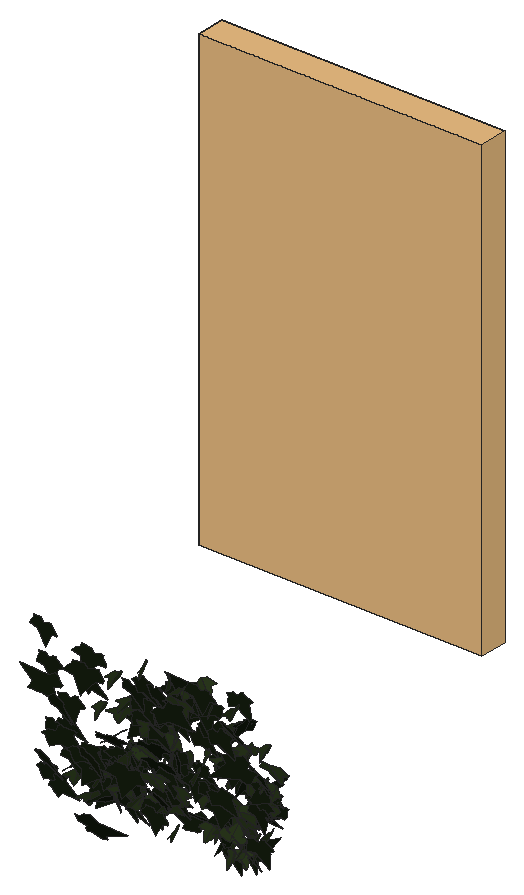
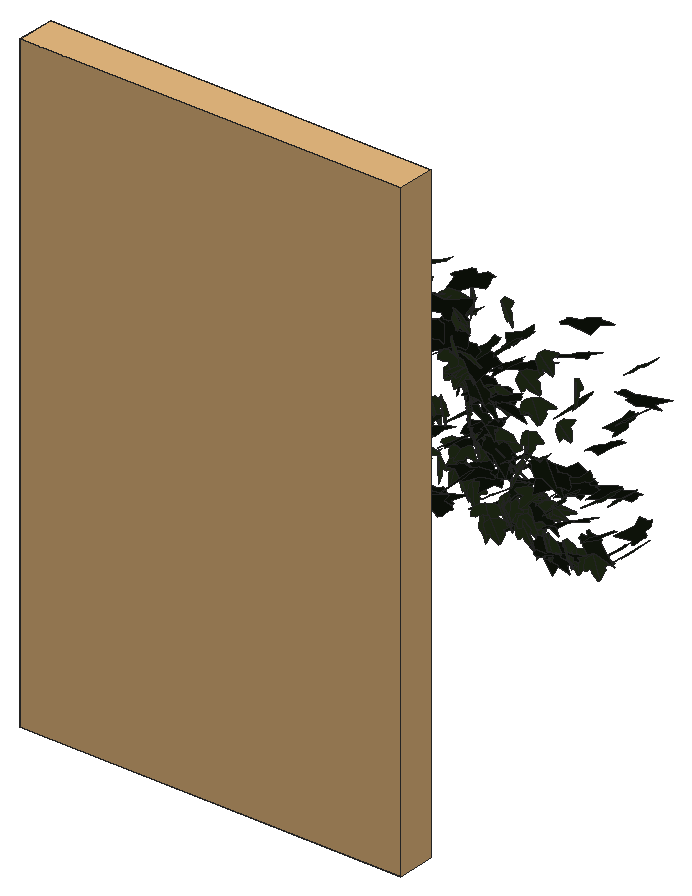
# SketchUp Ruby script. Lengths in millimetres.
U = 1.mm
M = Sketchup.active_model
def pt(a) = Geom::Point3d.new(a.map { |v| v * U })
def face(e, loops, mat)
  f = e.add_face(loops[0].map { |a| pt(a) })
  loops[1..].each { |l| e.add_face(l.map { |a| pt(a) }).erase! }
  f.material = f.back_material = mat if mat
  f
end
# faces: each face lists its corners as indices into pts; further lists are holes
def faces(e, pts, list, mat = nil) = list.each { |f| face(e, (f[0].is_a?(Array) ? f : [f]).map { |l| l.map { |i| pts[i] } }, mat) }
# xy, xz, yz: faces in a plane at the given z, y or x. An outline is a flat list of corners, or four numbers for a rectangle; further outlines are holes
def ring(l) = l.size == 4 ? [[l[0], l[1]], [l[2], l[1]], [l[2], l[3]], [l[0], l[3]]] : l.each_slice(2).to_a
def flat(e, list, mat, &to3) = list.each { |f| face(e, (f[0].is_a?(Array) ? f : [f]).map { |l| ring(l).map { |u, v| to3.(u, v) } }, mat) }
def xy(e, z, list, mat = nil) = flat(e, list, mat) { |x, y| [x, y, z] }
def xz(e, y, list, mat = nil) = flat(e, list, mat) { |x, z| [x, y, z] }
def yz(e, x, list, mat = nil) = flat(e, list, mat) { |y, z| [x, y, z] }
def lines(e, pts, list) = list.each { |a, b| e.add_line(pt(pts[a]), pt(pts[b])) }
# prism: a flat outline (further loops are holes) pulled along v
def prism(e, loops, v, mat = nil)
  f = face(e, loops, mat); d = Geom::Vector3d.new(v.map { |x| x * U })
  f.pushpull(f.normal.samedirection?(d) ? d.length : -d.length)
end
def box(e, o, s, mat = nil) = prism(e, [[o, [o[0] + s[0], o[1], o[2]], [o[0] + s[0], o[1] + s[1], o[2]], [o[0], o[1] + s[1], o[2]]]], [0, 0, s[2]], mat)
def at(x, y, z, deg = 0) = Geom::Transformation.translation(pt([x, y, z])) * Geom::Transformation.rotation(ORIGIN, Z_AXIS, deg.degrees)
def axes(o, x, y, z) = Geom::Transformation.new([*x, 0, *y, 0, *z, 0, *pt(o).to_a, 1])
def part(name) = M.definitions.add(name)
# library, detail: a bought-in or finely detailed component or shape, given as its bounding box
def library(name, o, s) = part(name).tap { |d| box(d.entities, o, s) }
def detail(e, o, s) = box(e.add_group.entities, o, s)
def put(e, d, t, mat = nil) = e.add_instance(d, t).tap { |i| i.material = mat if mat }
def group(e, t, mat = nil) = e.add_group.tap { |g| g.transformation = t; g.material = mat if mat }.entities
root = M.entities
M.materials.add("efeu1").color = [18, 25, 13]
M.materials.add("efeu2").color = [43, 57, 29]
c1 = part("ivyleaf_9")
p = [[39.1,54.8,31.7],[34.5,51.8,30.2],[-5.3,25.2,17.3],[-17.9,28.3,20.9],[-21.6,21.7,17],[-20.2,4.3,5.3],
  [-22.9,-0.3,2.5],[-17.1,-4,-0.6],[-2,-2.1,-1.2],[-0.7,-15.4,-10.1],[16.6,-22.3,-16.7],[21.1,-15.1,-12.5],
  [32.7,-10.7,-11],[46.1,-1.8,-6.6],[30.8,11.2,3.8]]
faces(c1.entities,p,[[0,1,2,3,4,5,6,7,8,9,10,11,12,13,14]],"efeu1")
c2 = library("ITDHP",[-33.4,-34.2,-15.9],[968.5,150,1668.6])
c3 = part("ivyleaf_10")
p = [[0,12.8,-0.8],[-1.5,51.3,-10.9],[-4.9,51,-11.6],[-13.6,26.5,-7.3],[-13.2,15.9,-4.6],[-21.1,19.3,-7.2],
  [-29.5,16.3,-8.3],[-29.2,8.3,-6.2],[-19.7,-9.8,0.5],[-7.6,-13,4],[1,-12.2,5.8],[-0.4,51.1,-11.1],
  [-1.5,51.1,-10.9],[1,-12.4,5.9],[16.9,-12.4,3.5],[35.1,9.1,-5.1],[35,12.9,-6.1],[20.5,16.4,-4.9],
  [15.8,15,-3.8],[15.3,27.6,-7.1],[12.8,31.3,-7.8]]
faces(c3.entities,p,[[0,1,2,3,4,5,6,7,8,9,10],[11,12,0,13,14,15,16,17,18,19,20]],"efeu2")
put(root,c1,axes([2483.7,708.7,4158.5],[-0.28262,-1.1774,0.40813],[0.0177,-0.41205,-1.18534],[2.37157,-0.13724,0.05748]))
put(root,c1,axes([2494.6,726.9,4001.3],[-0.09534,-1.22395,0.12593],[-0.03725,-0.12522,-1.22489],[2.34142,-0.05183,-0.01436]))
put(root,c1,axes([2497.5,675.4,3600.5],[1.44295,-0.99098,0.08108],[0.08914,-0.06625,-1.24774],[1.89024,0.75961,-0.00305]))
put(root,c1,axes([2509.6,688.7,3544.6],[0.92493,-1.0285,-0.50939],[-0.22035,0.50642,-1.13297],[2.17323,0.48908,0.10192]))
put(root,c1,axes([2529,725.7,3721.4],[0.20264,-1.17955,0.09647],[-0.00225,-0.09697,-1.18431],[2.25242,0.10602,-0.00986]))
put(root,c1,axes([2602.2,602.4,3970.9],[-2.12359,-0.52246,-0.45001],[-0.77802,-0.18816,1.23206],[-1.05684,1.18833,-0.00277]))
put(root,c2,axes([1909.4,2477.6,3547.4],[1.44679,0,0],[0,0.92467,0],[0,0,1.35933]))
put(root,c1,axes([2551.9,751.2,3734.9],[1.14067,-0.86466,-0.57736],[-0.1554,0.62522,-1.02109],[1.97265,0.54924,0.25342]))
put(root,c3,axes([2598.1,772.3,3510.4],[-0.90978,-1.05017,0.1465],[0.10312,-0.18468,-1.14708],[2.0154,-0.46461,0.12482]))
put(root,c1,axes([2583.1,773.7,3597.7],[-0.23495,-1.16003,-0.05168],[0.00538,0.05167,-1.16658],[2.20995,-0.12345,-0.00265]))
put(root,c1,axes([2565.9,687.9,3715.8],[0.15691,-0.76755,-1.00995],[0.83722,0.96657,-0.69868],[2.26442,-0.30418,0.32831]))
put(root,c1,axes([2622.7,769.4,3574.8],[-1.00385,0.89287,-0.49278],[0.22125,-0.49852,-1.02772],[-1.92828,-0.52202,0.13861]))
put(root,c1,axes([2581.8,662.6,3514.2],[1.14228,-0.69605,-0.86478],[-0.48035,0.87177,-0.87685],[2.05741,0.58998,0.27541]))
put(root,c1,axes([2607.7,714.6,3864.5],[-0.42573,-1.18321,-0.17776],[0.03449,0.17747,-1.20407],[2.27689,-0.22392,-0.015]))
put(root,c1,axes([2591,633.2,3904.1],[1.09347,-1.15014,0.0967],[0.0509,-0.09472,-1.28553],[2.19608,0.57487,-0.01835]))
put(root,c3,axes([2700.1,774.4,3522.2],[0.47999,-1.20059,-0.14065],[0.01719,0.14554,-1.22619],[2.30053,0.24941,0.03851]))
put(root,c3,axes([2704.2,721.3,3473.8],[-1.05201,-1.0084,-0.08689],[0.07914,0.07629,-1.14996],[1.92466,-0.55432,-0.00021]))
put(root,c3,axes([2704.1,724,4029.6],[0.45199,-1.14417,-0.40361],[0.25794,0.43371,-1.14976],[2.29463,0.17662,0.20875]))
put(root,c1,axes([2683.9,714.4,3985.6],[1.37408,-0.80214,-0.70953],[-0.53398,0.68414,-1.05894],[1.96698,0.74608,0.20819]))
put(root,c1,axes([2711.4,733.4,3584.4],[-1.23851,-0.88361,0.42411],[-0.16223,-0.45613,-1.08111],[1.85831,-0.62872,0.18828]))
put(root,c1,axes([2726.9,779,3484.5],[-1.55573,-0.74221,0.3045],[-0.29685,-0.27939,-1.09973],[1.4977,-0.82635,0.09833]))
put(root,c1,axes([2689.3,685.5,3685.3],[0.24428,-0.81486,-0.97339],[0.60001,0.96816,-0.76891],[2.34031,-0.16316,0.29873]))
put(root,c1,axes([2730.7,702.3,4114.1],[-1.33982,-0.9991,0.2392],[0.0036,-0.29123,-1.21086],[1.95522,-0.6841,0.16614]))
put(root,c1,axes([2762.3,783.8,3477.7],[-2.08455,-0.30009,-0.15658],[0.28567,0.0447,-1.13565],[0.5774,-1.10552,-0.00342]))
put(root,c3,axes([2749.9,733.1,3880.5],[-0.11071,-1.0711,0.57084],[0.28744,-0.57344,-1.06059],[2.29199,0.02018,0.16058]))
put(root,c1,axes([2722.9,682.6,3673.7],[0.50583,-1.1366,0.50822],[0.42371,-0.46791,-1.16288],[2.33139,0.33164,0.10108]))
put(root,c1,axes([2747.7,771.2,3575.9],[-0.74963,-1.0784,0.22297],[-0.00917,-0.23511,-1.14565],[2.0958,-0.38676,0.07474]))
put(root,c3,axes([2757.2,772.2,3518.6],[1.50085,-0.85793,-0.05577],[0.39331,0.26262,-1.11775],[1.58829,0.74567,0.32949]))
put(root,c1,axes([2757.5,751.7,3736],[2.10954,0.35329,-0.13884],[-0.29403,0.02844,-1.16103],[-0.6599,1.11671,0.0735]))
put(root,c1,axes([2756.1,763.9,3626.1],[0.16839,-1.11835,0.33834],[-0.00301,-0.33942,-1.12151],[2.22371,0.08423,-0.02714]))
put(root,c1,axes([2785.1,738.2,3482.9],[0.5915,1.09986,-0.06636],[-0.03875,-0.06321,-1.14292],[-2.0967,0.31145,0.0024]))
put(root,c3,axes([2814.5,741.1,3597.2],[0.70906,0.18084,1.13241],[-1.99432,-0.42999,0.41342],[0.88658,-1.11187,0.0243]))
put(root,c3,axes([2803.9,774.9,3610.7],[-0.50225,-0.39551,1.06163],[-1.11363,-0.88582,-0.47547],[1.8463,-0.64189,0.00201]))
put(root,c1,axes([2798.5,763.6,3752.1],[-0.61196,1.09711,-0.29601],[0.04604,-0.30096,-1.14171],[-2.16219,-0.31692,0.05947]))
put(root,c3,axes([2778.8,773,3522.3],[0.93965,-1.03052,-0.18486],[0.04886,0.21624,-1.13688],[1.992,0.4808,0.11509]))
put(root,c1,axes([2759.2,765.2,3665.7],[0.44507,-1.144,-0.19589],[-0.10287,0.18888,-1.16756],[2.20655,0.23955,-0.01492]))
put(root,c1,axes([2804,771.2,3617.7],[-0.76561,0.92276,-0.5849],[0.50641,-0.52177,-1.00617],[-2.01667,-0.48134,-0.03061]))
put(root,c3,axes([2804.2,742,3624.3],[-1.56209,0.76875,-0.31185],[0.22143,-0.32768,-1.114],[-1.56328,-0.81458,0.15382]))
put(root,c3,axes([2814.1,739.5,3484.2],[-0.97729,1.01183,0.15132],[-0.1744,0.12315,-1.13438],[-1.9393,-0.52098,0.02576]))
put(root,c1,axes([2814.3,559.7,4134.4],[-1.51316,-1.08884,-0.15786],[0.17728,0.12745,-1.34822],[2.08643,-0.8005,0.00007]))
put(root,c3,axes([2843.6,704.8,4062.4],[-0.2297,-1.12356,0.51681],[0.12774,-0.52445,-1.12449],[2.35026,-0.0813,0.11163]))
put(root,c3,axes([2832.6,750.7,3633.8],[-2.07695,0.19974,-0.3925],[0.74315,-0.04621,-1.10918],[-0.38763,-1.15881,-0.02342]))
put(root,c3,axes([2859.1,735.1,3539.4],[-1.60311,-0.73608,0.27744],[-0.27349,-0.25565,-1.11458],[1.47192,-0.84919,0.09506]))
put(root,c3,axes([2877,757.9,3515.9],[-1.09185,0.39819,0.94383],[-1.63681,0.40048,-0.69171],[-1.05919,-1.02935,0.09599]))
put(root,c1,axes([2853.7,756.2,3681.8],[-1.6214,-0.82503,0.11182],[0.17638,-0.25297,-1.16034],[1.5747,-0.82116,0.24511]))
put(root,c3,axes([2868.7,715.3,3908.1],[-1.30452,-0.99741,0.17976],[-0.06083,-0.19564,-1.20734],[1.92789,-0.68108,0.08355]))
put(root,c1,axes([2862.9,770.4,3652.8],[0.95651,-0.84126,-0.63918],[-0.53265,0.57652,-0.97885],[1.93896,0.57338,0.04641]))
put(root,c3,axes([2878.5,765.8,3718],[-0.68602,0.81326,0.77222],[0.61912,-0.70043,0.8895],[2.04264,0.48543,-0.01025]))
put(root,c3,axes([2884.6,765.1,3703.9],[-0.69273,1.11877,0.07061],[-0.05026,0.06566,-1.17648],[-2.13288,-0.36491,0.00479]))
put(root,c1,axes([2903.7,716.4,3643.8],[-1.64804,-0.65817,0.41688],[-0.28647,-0.47021,-1.05502],[1.45483,-0.83817,0.26451]))
put(root,c3,axes([2913.3,698.4,3972.1],[-0.49704,-1.05133,0.58337],[-0.23645,-0.57019,-1.08318],[2.27605,-0.28882,0.01487]))
put(root,c1,axes([2880.3,679.8,3699.3],[0.84745,-1.04105,-0.37356],[0.0111,0.4049,-1.12144],[2.10499,0.41698,0.15631]))
put(root,c1,axes([2886.1,700.3,3533],[0.74726,-1.09628,0.11826],[0.06322,-0.11372,-1.16445],[2.0976,0.39397,-0.00703]))
put(root,c1,axes([2913.3,759.2,3728],[-0.31504,-1.16069,0.13177],[-0.05045,-0.12932,-1.17241],[2.22265,-0.16745,-0.00793]))
put(root,c1,axes([2899.5,706.8,3509.4],[1.45235,-0.82894,-0.30772],[-0.18451,0.32558,-1.11748],[1.67269,0.75566,0.14392]))
put(root,c3,axes([2929.8,768.5,3557.7],[0.89543,-1.0577,-0.09463],[-0.02823,0.09695,-1.15734],[2.02087,0.47002,0.02576]))
put(root,c3,axes([2931.4,657.2,3752.6],[-0.45827,-1.11207,-0.41383],[0.23429,0.39658,-1.13732],[2.24609,-0.26826,0.0342]))
put(root,c3,axes([2934.2,750.2,3709.9],[0.69374,-1.07837,-0.26785],[0.05338,0.29074,-1.13234],[2.11404,0.34654,0.11649]))
put(root,c1,axes([2913,745.4,3688.5],[0.7813,-1.10678,-0.05108],[-0.04257,0.04619,-1.18045],[2.10823,0.4111,-0.0049]))
put(root,c1,axes([2920.1,723.7,3594],[-0.39788,-0.73732,0.96269],[0.30302,-0.98512,-0.71993],[2.28785,0.00225,0.26278]))
put(root,c3,axes([2940.6,727.2,3556.9],[-0.2647,-1.01817,-0.53863],[0.27941,0.52245,-1.02549],[2.17435,-0.19108,0.06621]))
put(root,c3,axes([2932.7,695.6,3508.5],[-0.39581,-1.05143,0.59792],[0.18737,0.58997,1.07169],[-2.29438,0.22956,-0.01563]))
put(root,c1,axes([2972.7,739.9,3724],[-1.82693,0.67363,-0.119],[0.17244,-0.07804,-1.17265],[-1.29044,-0.96412,0.01177]))
put(root,c1,axes([2961.1,757.5,3756.4],[0.14987,1.18539,0.08268],[0.0011,0.08282,-1.18799],[-2.26151,0.0786,0.0049]))
put(root,c1,axes([2967.5,737.8,3881.3],[-2.19838,-0.31213,-0.1349],[0.29087,-0.04986,-1.19333],[0.5781,-1.16188,0.08745]))
put(root,c3,axes([2958.3,734.8,3564.9],[-0.06315,-1.14737,0.18508],[0.03487,-0.18565,-1.14761],[2.21162,-0.02984,0.02338]))
put(root,c1,axes([2899.2,468.3,3514.5],[0.73027,-0.27467,1.40411],[2.23565,-0.76942,-0.47152],[1.55446,1.23562,0.01851]))
put(root,c1,axes([2921.2,762.2,3703.4],[0.86558,-0.0989,-1.08639],[1.98527,-0.30502,0.46446],[-0.60756,-1.13756,-0.03009]))
put(root,c3,axes([2974.8,770.9,3497],[-0.92703,-1.02703,0.27994],[0.01351,-0.31098,-1.12857],[2.02592,-0.46788,0.13562]))
put(root,c1,axes([2958.4,734.5,3908.7],[-0.06841,-1.03805,-0.60014],[0.13413,0.59755,-1.03778],[2.27809,-0.06636,0.04308]))
put(root,c1,axes([2959.9,715.2,4065.6],[0.8788,-1.11229,-0.30252],[-0.11876,0.30129,-1.20302],[2.19059,0.46255,0.05614]))
put(root,c3,axes([2993.8,782.6,3506.8],[-0.22074,-1.09817,-0.32836],[0.04212,0.32783,-1.10421],[2.18105,-0.11747,-0.01191]))
put(root,c1,axes([2961.5,661.8,4066.1],[0.24655,-1.19611,0.4608],[0.32641,-0.4428,-1.19763],[2.41759,0.18177,0.1147]))
put(root,c1,axes([2973.2,699.5,3997.5],[0.21639,-1.16031,-0.39927],[-0.09337,0.39636,-1.16583],[2.33353,0.12346,-0.00962]))
put(root,c3,axes([2949.3,718.9,3757.7],[1.06799,0.12187,1.09187],[2.04625,0.19124,-0.57392],[-0.43004,1.21264,-0.01922]))
put(root,c1,axes([2981.1,747.7,3822],[0.56611,-0.78401,-0.84788],[-0.52285,0.80237,-0.83831],[2.13472,0.40444,0.01952]))
put(root,c3,axes([3002.6,766.3,3538.5],[-1.5935,-0.80292,0.19809],[0.0782,-0.32193,-1.1312],[1.57199,-0.79789,0.25707]))
put(root,c3,axes([3026.9,697.4,3885.4],[-1.96171,-0.03764,0.63935],[-1.20301,-0.13529,-1.02702],[0.19629,-1.20536,0.0953]))
put(root,c3,axes([3000.8,681.4,4166.9],[0.53831,-1.20646,0.1928],[0.12603,-0.18247,-1.23896],[2.32185,0.28962,0.02255]))
put(root,c1,axes([3024.8,750.6,3836.3],[-0.24771,1.01193,0.63516],[-0.24591,0.62325,-1.01943],[-2.26051,-0.17869,0.0413]))
put(root,c1,axes([3036.6,738.5,3916],[0.16615,0.75209,0.94289],[-0.12967,0.94692,-0.749],[-2.29179,0.00095,0.11074]))
put(root,c1,axes([3002.6,752.3,3816.5],[-0.00914,-1.05681,-0.56667],[0.11862,0.56569,-1.05551],[2.27914,-0.03368,0.05266]))
put(root,c1,axes([3054.8,740.2,3906.8],[-0.65141,1.1467,0.01347],[-0.15579,-0.01041,-1.19392],[-2.17699,-0.34238,0.08141]))
put(root,c1,axes([3015.4,732.5,3533.5],[-0.41656,-1.12441,-0.29998],[0.18174,0.28686,-1.14489],[2.20735,-0.23581,0.03766]))
put(root,c1,axes([3059.3,693.4,3748.8],[1.51437,0.51951,-0.76299],[-1.33216,-0.3171,-0.94588],[-1.14526,1.05581,0.09134]))
put(root,c3,axes([3055.3,757.8,3757.5],[0.63119,-1.07137,-0.3998],[-0.18744,0.38797,-1.12136],[2.16829,0.34542,0.01945]))
put(root,c1,axes([3024.2,722.8,4043],[0.84762,-1.1524,0.09873],[-0.00353,-0.10651,-1.23482],[2.20128,0.44357,-0.04]))
put(root,c1,axes([3032.5,740.9,3877.3],[0.2122,-1.18236,-0.20142],[-0.06185,0.19924,-1.18753],[2.28185,0.11535,-0.01346]))
put(root,c3,axes([3045.4,674.6,3691.8],[-2.1752,-0.2646,-0.40805],[0.76238,0.07879,-1.17308],[0.52487,-1.21101,0.01284]))
put(root,c1,axes([3060,721.4,4011.8],[1.6934,0.76933,-0.3742],[-0.68532,-0.15296,-1.17069],[-1.47694,0.95305,0.11418]))
put(root,c1,axes([3048.7,680.6,3612.5],[2.19592,-0.1851,-0.55266],[-1.02994,0.11494,-1.16829],[0.41191,1.27416,0.0251]))
put(root,c1,axes([3054.5,684.9,3526.2],[-0.46488,-1.11693,0.32571],[0.0361,-0.33659,-1.14001],[2.21398,-0.22904,0.08698]))
put(root,c1,axes([3065.5,634.2,3856.9],[2.02974,0.46332,-0.34294],[-0.57804,-0.16134,-1.1625],[-0.93243,1.10859,-0.02586]))
put(root,c1,axes([3059.5,711.7,3888.8],[-0.03345,-1.11727,-0.50146],[0.03894,0.50117,-1.11735],[2.33042,-0.02441,0.01147]))
put(root,c3,axes([3081.7,724,3559.2],[-0.22418,-1.13347,-0.34215],[0.14668,0.33577,-1.13886],[2.24858,-0.13491,0.04018]))
put(root,c1,axes([3089.1,727.4,3622.8],[-1.11889,-0.80601,-0.62732],[0.82414,0.45885,-0.99537],[1.76052,-0.72706,0.06726]))
put(root,c3,axes([3104.4,719.4,3883],[1.35242,-0.9389,-0.27094],[-0.0111,0.33092,-1.16205],[1.8598,0.68473,0.19009]))
put(root,c1,axes([3097.8,732.7,3604.8],[1.10962,-0.41374,-0.93092],[-0.74195,0.90034,-0.6443],[1.79125,0.62923,0.3098]))
put(root,c3,axes([3103.5,739.4,3946.1],[0.72448,1.0859,0.39605],[0.02061,0.41361,-1.14445],[-2.19976,0.36151,0.11971]))
put(root,c3,axes([3120.4,747,3989.5],[-2.23402,-0.28732,0.00456],[-0.01287,0.00845,-1.20844],[0.54674,-1.1738,-0.00982]))
put(root,c1,axes([3111.1,444.9,3837.1],[-1.27381,-1.27237,0.04912],[-0.00129,-0.05514,-1.43745],[2.42338,-0.66883,0.02506]))
put(root,c1,axes([3107.4,719.8,3708.5],[-0.67556,-1.13337,-0.22129],[0.14261,0.20841,-1.18762],[2.19312,-0.36267,0.00906]))
put(root,c3,axes([3129.4,749.2,3946.9],[-1.17939,-0.94713,0.40045],[-0.09752,-0.43852,-1.11647],[1.95464,-0.59336,0.18592]))
put(root,c1,axes([3120.7,751.1,3791.8],[-0.68724,-0.96355,0.6098],[-0.12515,-0.62099,-1.02016],[2.16661,-0.3415,0.1345]))
put(root,c1,axes([3105.3,737.9,3953.8],[0.47691,-1.157,-0.28827],[0.00078,0.29465,-1.18225],[2.26932,0.24305,0.06099]))
put(root,c1,axes([3118.4,765.9,3709.4],[-0.57199,-1.07879,0.36576],[0.00718,-0.37921,-1.11538],[2.16794,-0.28337,0.1002]))
put(root,c3,axes([3131.4,669.3,4153.6],[0.70664,-1.07508,-0.53467],[0.18068,0.58418,-1.10871],[2.278,0.28716,0.25379]))
put(root,c3,axes([3130.7,699.6,3874.4],[1.97237,-0.5924,-0.11984],[-0.11988,0.13072,-1.1909],[1.14403,1.03503,0.08182]))
put(root,c3,axes([3133.7,688.7,3805.2],[0.89338,-1.00167,-0.43361],[0.03202,0.47859,-1.08737],[2.07709,0.42345,0.20326]))
put(root,c1,axes([3115.6,765.4,3723.1],[-0.00565,-1.17707,-0.08101],[-0.00083,0.08101,-1.17707],[2.2455,-0.00293,-0.00064]))
put(root,c3,axes([3141.9,699.4,3883.9],[0.96579,-1.07227,-0.18734],[-0.17822,0.16292,-1.18619],[2.06397,0.51581,-0.01476]))
put(root,c1,axes([3131,733,3984.9],[-0.64457,-1.09804,0.41733],[-0.00809,-0.43318,-1.14319],[2.23561,-0.31815,0.11619]))
put(root,c3,axes([3144.5,730.4,4022.2],[0.41447,-1.1235,0.44119],[0.17445,-0.43162,-1.14439],[2.29057,0.23617,0.00733]))
put(root,c3,axes([3153.2,707.7,4095.6],[0.04137,-1.15734,0.43482],[0.02149,-0.43468,-1.15754],[2.35289,0.02432,0.00293]))
put(root,c3,axes([3149.5,696.2,3663.5],[-2.15335,0.26491,-0.24577],[0.43342,-0.10447,-1.16101],[-0.53397,-1.1531,0.04872]))
put(root,c1,axes([3130.8,703.8,3627],[0.91314,-1.0469,-0.22332],[-0.12086,0.21646,-1.15116],[2.03369,0.48293,0.03186]))
put(root,c1,axes([3145.8,695.1,4092.5],[-0.55824,-1.08127,0.51387],[0.09305,-0.53945,-1.10718],[2.27655,-0.24309,0.17126]))
put(root,c3,axes([3168.8,773.1,3638.4],[0.30687,-0.95516,-0.63787],[0.01117,0.6448,-0.96406],[2.18593,0.1308,0.09448]))
put(root,c1,axes([3196.8,722.2,4099.9],[0.73495,0.00991,1.17737],[-2.222,0.16357,0.38156],[-0.28998,-1.22824,0.06031]))
put(root,c3,axes([3167.7,695.3,3596.6],[-0.72725,-1.06188,-0.52427],[0.45264,0.47085,-1.12703],[2.20794,-0.44629,0.05837]))
put(root,c1,axes([3184.8,725.9,4057.2],[0.19533,1.11082,-0.52236],[-0.09389,-0.52003,-1.11555],[-2.3343,0.11387,0.00116]))
put(root,c1,axes([3209.3,758,3495.8],[-0.31649,0.45298,1.04351],[-2.16257,-0.11656,-0.13048],[0.10351,-1.05023,0.46456]))
put(root,c1,axes([3156.7,722.5,4050.5],[1.82604,0.73595,0.21965],[0.36375,0.11164,-1.2089],[-1.41573,0.97793,-0.02729]))
put(root,c3,axes([3170,705.6,4105.4],[1.82032,-0.74795,0.22627],[0.2901,-0.17218,-1.21349],[1.45865,0.96765,-0.04103]))
put(root,c3,axes([3185.5,644.6,3515.8],[0.25766,-1.15524,-0.12506],[-0.02427,0.12442,-1.16315],[2.21137,0.13597,0.00181]))
put(root,c3,axes([3191.6,730.6,3804],[1.05514,-1.03296,-0.29326],[0.06553,0.34697,-1.15706],[2.04257,0.52247,0.18861]))
put(root,c1,axes([3162.3,772.1,3511.4],[2.01088,-0.05098,0.50818],[0.97129,0.05974,-1.05508],[0.038,1.17092,0.07596]))
put(root,c3,axes([3212.3,628.9,4099.1],[-2.28867,0.27266,-0.15968],[0.29431,-0.04009,-1.23305],[-0.52442,-1.21243,0.00486]))
put(root,c1,axes([3200.4,640.2,3835.9],[0.24859,-0.31132,-1.225],[1.92708,-0.71132,0.28874],[-1.43976,-1.00584,0.17496]))
put(root,c1,axes([3201.2,767.7,3753.4],[1.08844,-0.99368,-0.26786],[-0.00921,0.30384,-1.13749],[1.95867,0.55363,0.1435]))
put(root,c1,axes([3231.8,739.5,3710.1],[-0.95102,-1.07408,0.06515],[-0.01373,-0.06848,-1.18442],[2.0479,-0.49925,0.02231]))
put(root,c3,axes([3249.4,699,3767],[0.3438,-1.20547,-0.05667],[-0.00444,0.05695,-1.21892],[2.29678,0.18055,0.00612]))
put(root,c3,axes([3270.2,755.8,3642.9],[-1.98756,-0.39407,0.41704],[-0.57663,-0.35673,-1.0958],[0.92734,-1.06643,0.21245]))
put(root,c1,axes([3234.7,524.8,4121.2],[0.171,-0.64685,-1.26838],[0.02637,1.27124,-0.64732],[2.70965,0.02845,0.08634]))
put(root,c1,axes([3244.1,709.9,3936.8],[0.84095,-1.01629,-0.53112],[-0.06635,0.55702,-1.09484],[2.1814,0.40873,0.17145]))
put(root,c1,axes([3271.3,684.8,4070.8],[-0.66304,-0.90881,0.76609],[-0.54288,-0.71107,-0.97325],[2.19609,-0.45017,-0.00929]))
put(root,c3,axes([3274.9,775.7,3510.9],[-0.69254,-1.02386,-0.3654],[0.2686,0.33758,-1.08643],[2.05148,-0.38983,0.0189]))
put(root,c1,axes([3296.6,732,3684.2],[1.18515,0.33075,-0.97016],[-1.93281,0.04545,-0.63636],[-0.26403,1.15192,0.30367]))
put(root,c3,axes([3268.3,715,4169.5],[0.40489,1.2267,0.08282],[0.07618,0.0771,-1.24474],[-2.33874,0.21488,-0.02621]))
put(root,c3,axes([3283.3,739.2,3516.3],[1.87527,-0.69641,-0.01824],[-0.03911,0.00252,-1.20655],[1.32528,0.98549,-0.0098]))
put(root,c1,axes([3269,728.9,3970.7],[0.99057,-1.05811,-0.30369],[-0.09329,0.31331,-1.17565],[2.09301,0.51474,0.09133]))
put(root,c1,axes([3282.7,731.5,3701.2],[0.20315,-1.18347,-0.07002],[-0.02591,0.06907,-1.18825],[2.25617,0.10735,-0.00734]))
put(root,c3,axes([3315.2,679.9,3878.4],[0.67324,-1.15693,-0.2481],[-0.12961,0.23861,-1.20979],[2.2482,0.36021,0.00455]))
put(root,c3,axes([3306.1,768,3478.3],[-1.26858,0.95154,-0.11806],[0.15281,-0.08788,-1.16168],[-1.81845,-0.67119,-0.01526]))
put(root,c1,axes([3326.3,694.2,4103.7],[-1.81374,-0.68747,0.39775],[-0.33725,-0.42158,-1.15321],[1.47351,-0.9427,0.22566]))
put(root,c1,axes([3345.7,788.2,3566.8],[-2.16089,0.01597,0.18946],[-0.3601,0.01832,-1.13541],[-0.03572,-1.15095,-0.01544]))
put(root,c1,axes([3303.3,678.2,4079.5],[-0.18148,-1.22202,0.15335],[0.03797,-0.15533,-1.22532],[2.34368,-0.09211,0.03173]))
put(root,c3,axes([3321.3,693.4,4088.3],[0.59222,-1.09953,-0.51575],[0.18641,0.55339,-1.12069],[2.30387,0.23786,0.22325]))
put(root,c3,axes([3323.5,748,3523.5],[0.25396,-1.06932,0.45628],[0.33602,-0.43532,-1.07181],[2.187,0.19105,0.11169]))
put(root,c1,axes([3313.6,637.4,4180.7],[-0.57406,-1.17771,0.26312],[0.40199,-0.31856,-1.18369],[2.26122,-0.24235,0.27723]))
put(root,c1,axes([3345.7,749.2,3830.8],[-0.6805,-0.99389,0.54034],[-0.24244,-0.52771,-1.05495],[2.13935,-0.37594,0.05232]))
put(root,c3,axes([3370.6,727.9,3848.2],[-1.21707,-0.84249,0.57455],[-0.31164,-0.58454,-1.03939],[1.91561,-0.63036,0.19594]))
put(root,c3,axes([3362.8,746.9,3675.7],[0.21283,-1.10768,0.4077],[0.03067,-0.40806,-1.11307],[2.2462,0.11053,-0.02343]))
put(root,c1,axes([3393.7,746,3586.2],[-0.17161,0.24721,-1.19825],[-2.22925,0.32966,0.15615],[0.67269,1.15553,0.2118]))
put(root,c1,axes([3364.8,743.5,3979.5],[-0.68973,-1.09574,0.35859],[-0.00103,-0.37572,-1.14865],[2.19424,-0.34461,0.11218]))
put(root,c3,axes([3381.3,773.9,3480.8],[0.03838,-1.1673,-0.03753],[-0.01554,0.03739,-1.16745],[2.2227,0.02042,-0.00752]))
put(root,c1,axes([3405.6,702,3535],[-1.56897,0.49475,-0.73156],[1.08973,-0.4625,-0.95802],[-1.27969,-1.00044,0.08111]))
put(root,c3,axes([3403.1,703,3775.5],[0.43006,-0.48447,1.12183],[-0.66862,1.06693,0.53152],[-2.22748,-0.41379,0.05705]))
put(root,c3,axes([3413.8,723.3,3591.6],[0.62498,-0.97487,-0.56849],[-0.24775,0.55539,-1.0276],[2.13345,0.35008,0.0472]))
put(root,c1,axes([3402.7,672.3,3686],[-0.99379,-1.08101,-0.06386],[0.03673,0.06159,-1.20048],[2.06063,-0.52244,-0.0094]))
put(root,c3,axes([3393.6,730,3689.7],[-1.65511,0.69627,-0.46587],[0.74726,-0.25442,-1.1132],[-1.40845,-0.9532,-0.04317]))
put(root,c1,axes([3378.3,735,3541.3],[0.40908,-0.76707,0.87556],[0.57154,-0.82368,-0.79534],[2.14041,0.36654,0.04504]))
put(root,c1,axes([3383.3,757.3,3518.4],[0.8639,-1.08437,0.1036],[0.07858,-0.09503,-1.17554],[2.07167,0.45579,0.00138]))
put(root,c1,axes([3439.8,728.2,3656.4],[1.1836,0.35974,-1.02332],[-1.84175,-0.3489,-0.71075],[-0.93264,1.14552,0.10489]))
put(root,c1,axes([3410.3,722.4,3839.6],[-0.64556,-1.08928,0.3941],[0.13114,-0.4289,-1.12614],[2.20072,-0.29397,0.18271]))
put(root,c3,axes([3429.6,704.3,4040.8],[-0.39132,-1.21741,0.16391],[-0.00587,-0.16567,-1.23441],[2.33787,-0.20419,0.02434]))
put(root,c3,axes([3425.6,776.9,3564.3],[-1.94238,0.51251,-0.21088],[0.23048,-0.22499,-1.13289],[-1.02927,-1.01757,0.14428]))
put(root,c1,axes([3403.5,641.2,3756.4],[0.43795,-1.06456,-0.52231],[0.25185,0.55179,-1.06633],[2.24269,0.14592,0.22174]))
put(root,c3,axes([3445.2,728.6,3549.6],[1.03819,-1.03915,-0.18769],[-0.16996,0.1651,-1.17362],[2.00251,0.55275,-0.0023]))
put(root,c3,axes([3429,687.2,3550.1],[2.23136,0.25903,-0.33483],[0.6221,0.0726,1.2007],[0.51198,-1.21714,0.00036]))
put(root,c1,axes([3426.2,697.4,3481.8],[0.22561,-1.13736,0.27835],[0.15318,-0.2712,-1.14241],[2.22324,0.1341,0.05046]))
put(root,c1,axes([3431,727.3,4156.6],[0.26485,-1.16899,-0.36772],[-0.02412,0.36869,-1.17687],[2.33216,0.13657,0.02959]))
put(root,c3,axes([3449.1,699.3,3948.9],[-0.04869,-1.09118,-0.55827],[0.53237,0.53845,-1.06527],[2.27118,-0.14961,0.23773]))
put(root,c3,axes([3466.6,745.6,3592.3],[-1.44144,0.80985,0.30465],[-0.48296,0.17917,-1.10716],[-1.57434,-0.79645,0.06071]))
put(root,c3,axes([3455.6,652.7,3498.9],[1.33709,-0.9017,0.30657],[0.35736,-0.24234,-1.14308],[1.77702,0.72721,-0.00079]))
put(root,c3,axes([3475.3,643.1,4155.7],[-0.29245,-1.25855,-0.09653],[-0.00339,0.09746,-1.26782],[2.4023,-0.15307,-0.01354]))
put(root,c3,axes([3453.3,691,3484.8],[1.11737,0.98322,0.40408],[0.37214,0.35385,-1.14509],[-1.9886,0.61868,0.01276]))
put(root,c3,axes([3478.9,714.8,3507.2],[0.04188,0.66275,-1.06763],[-0.70005,-1.01762,-0.6393],[-2.28683,0.32365,0.17615]))
put(root,c1,axes([3483.9,718.2,3643.2],[-0.10858,-0.05588,1.254],[0.80249,1.1815,0.07183],[-2.25017,0.42406,-0.03489]))
put(root,c3,axes([3486.2,764.4,3539],[-0.21048,-1.09252,0.37054],[0.08646,-0.37607,-1.09528],[2.19392,-0.09,0.07871]))
put(root,c1,axes([3464.4,757.5,3473],[0.11746,-1.14293,0.20643],[0.02654,-0.20597,-1.14459],[2.21026,0.06321,0.00278]))
put(root,c1,axes([3449.3,628,4074.1],[1.82275,-0.91663,0.09489],[0.15505,-0.0521,-1.32556],[1.74699,0.961,0.01864]))
put(root,c1,axes([3484.1,715.4,3812.4],[-0.36822,0.04003,-1.17983],[1.26923,-0.98281,-0.14271],[-1.85388,-0.68082,0.13663]))
put(root,c1,axes([3456.1,743.2,3481],[0.67163,-0.95674,0.57398],[0.45329,-0.52353,-1.01909],[2.07447,0.42415,0.03685]))
put(root,c1,axes([3500.6,688.5,4081.3],[-0.33109,0.73755,-1.01767],[0.54603,-0.97694,-0.75708],[-2.32885,-0.33391,-0.03283]))
put(root,c3,axes([3501.3,705.4,3961.2],[-1.16924,-0.99369,0.40384],[-0.15012,-0.42228,-1.15905],[2.03588,-0.60183,0.14647]))
put(root,c3,axes([3493.7,722.8,3948.5],[0.54873,-1.16287,-0.21213],[0.03053,0.22217,-1.19615],[2.24948,0.28065,0.06798]))
put(root,c3,axes([3451,723.2,3633.3],[-0.18869,0.01628,-1.24758],[1.85467,-0.78052,-0.08762],[-1.48286,-0.9783,0.04915]))
put(root,c1,axes([3466.3,559.5,4078.7],[0.4934,-1.17083,-0.34469],[0.07169,0.35989,-1.19412],[2.32177,0.2377,0.11012]))
put(root,c1,axes([3503.5,687.5,4084],[-0.60279,0.63119,-1.05487],[0.86325,-0.95246,-0.7061],[-2.17451,-0.55308,0.01211]))
put(root,c3,axes([3509.4,704.5,3786.2],[-2.18147,0.3522,0.17655],[-0.43284,-0.14802,-1.18126],[-0.61226,-1.15024,0.20607]))
put(root,c1,axes([3482.2,733.6,3783.1],[-0.28586,-1.08353,-0.52219],[0.44691,0.4897,-1.08367],[2.24512,-0.23544,0.14923]))
put(root,c1,axes([3520.8,776.6,3615.4],[0.38035,1.1489,0.00557],[-0.05855,0.011,-1.16571],[-2.18583,0.19962,0.03219]))
put(root,c3,axes([3540.4,703.8,3822.2],[1.40941,-0.58601,-0.82168],[-1.18815,0.53479,-0.94405],[1.50921,0.96828,0.02413]))
put(root,c1,axes([3494.3,749.9,3658],[2.209,0.13063,0.24963],[0.48028,-0.01145,-1.16736],[-0.23844,1.18716,-0.03873]))
put(root,c3,axes([3529.2,727.3,3518],[0.63425,-0.98199,0.59413],[0.41109,-0.55396,-1.03675],[2.14534,0.39646,0.02301]))
put(root,c1,axes([3517.2,719.3,3510.6],[-0.30734,-0.03357,1.25588],[2.21227,0.47642,0.1622],[-0.90718,1.17318,-0.02993]))
put(root,c1,axes([3585.8,574.7,3959.7],[-2.56302,-0.23569,0.48348],[-0.89295,-0.1226,-1.36664],[0.50053,-1.42559,0.0376]))
put(root,c3,axes([3513.4,672.3,3695.5],[0.53763,-0.11424,-1.22465],[2.12802,-0.49967,0.30453],[-0.9753,-1.15321,-0.01063]))
put(root,c3,axes([3593.4,731.6,3726],[0.9001,0.02208,-1.06905],[-1.70976,0.64218,-0.38417],[1.1037,0.97681,0.27673]))
put(root,c1,axes([3557.3,733.2,3737.4],[-0.95839,-1.04626,0.29042],[-0.07569,-0.30215,-1.15746],[2.06515,-0.49662,0.09236]))
put(root,c3,axes([3571.5,717.1,3830.7],[0.47457,-1.14895,0.25092],[0.12138,-0.24291,-1.17565],[2.23492,0.25716,0.01057]))
put(root,c3,axes([3571.9,723.9,3981.4],[-0.03493,-1.08463,0.54593],[0.25719,-0.54442,-1.0771],[2.29665,0.04447,0.12892]))
put(root,c3,axes([3577.9,737.8,3599.7],[0.07298,-1.17333,0.0616],[-0.01472,-0.06189,-1.17392],[2.23611,0.03788,-0.00974]))
put(root,c1,axes([3594.3,769.9,3709.5],[-2.21642,-0.061,-0.17261],[0.32889,0.00067,-1.16614],[0.11503,-1.1773,0.00828]))
put(root,c1,axes([3547.2,683.1,3885.9],[1.00993,-0.99909,0.44125],[0.37449,-0.39509,-1.13122],[2.04464,0.56585,-0.01076]))
put(root,c1,axes([3608.9,709,3805.4],[-1.92523,-0.58175,0.34738],[-0.56836,-0.17751,-1.16692],[1.15755,-1.05473,0.00479]))
put(root,c1,axes([3573.4,675.4,3578.1],[0.02621,-1.18213,-0.28498],[0.08325,0.2853,-1.18133],[2.31279,0.00312,0.04575]))
put(root,c1,axes([3574.3,716.1,3826.2],[1.35551,-0.94681,-0.23207],[-0.30133,0.17125,-1.18456],[1.83068,0.72925,-0.02314]))
put(root,c1,axes([3588,661.1,3735.2],[-0.03299,-1.15,0.38369],[0.08971,-0.38408,-1.14904],[2.30555,-0.00151,0.0502]))
put(root,c1,axes([3640.4,730.7,3849.4],[-1.28353,0.99577,-0.21635],[0.12154,-0.21764,-1.20073],[-1.93555,-0.67399,0.06808]))
put(root,c3,axes([3624.6,694.6,3924.7],[-2.26783,0.27243,-0.25757],[0.48415,-0.04291,-1.22225],[-0.52415,-1.21835,-0.01455]))
put(root,c3,axes([3624,699.8,3829.1],[1.79745,-0.74722,0.2022],[0.31668,-0.11555,-1.20422],[1.43881,0.9589,0.01245]))
